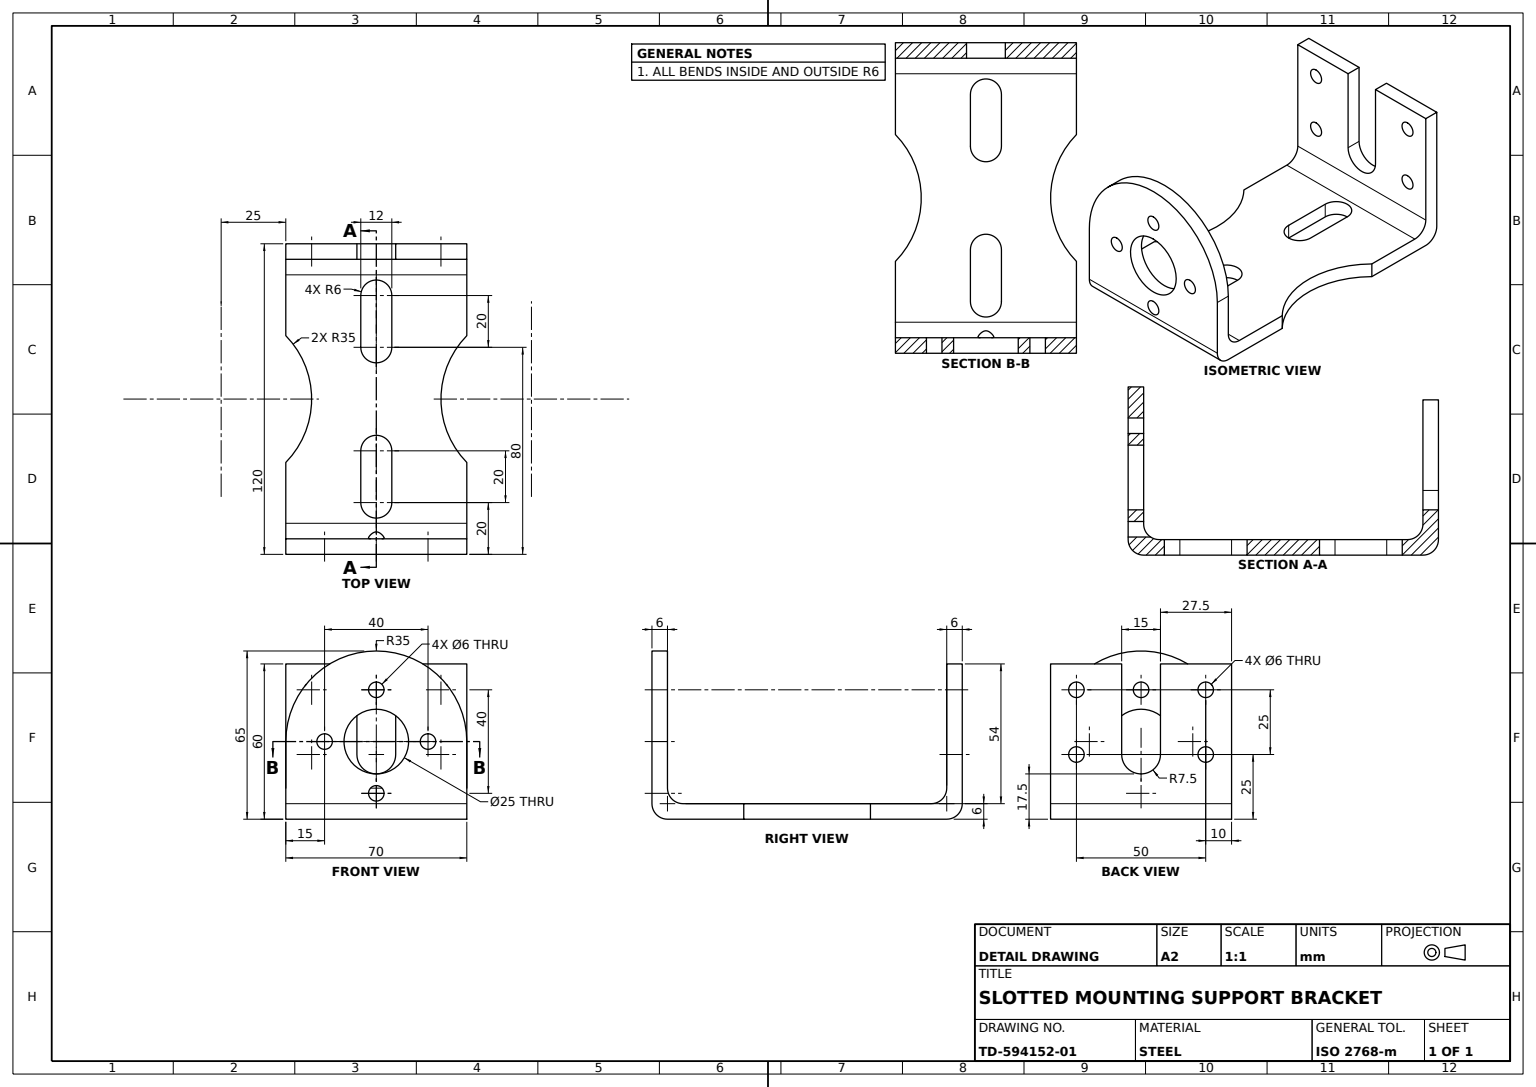
ISO-10303-21;
HEADER;
FILE_DESCRIPTION((''),'2;1');
FILE_NAME('','',(''),(''),'','','');
FILE_SCHEMA(('AUTOMOTIVE_DESIGN'));
ENDSEC;
DATA;
#1=APPLICATION_CONTEXT('');
#2=PRODUCT_CONTEXT('',#1,'mechanical');
#3=PRODUCT('','','',(#2));
#4=PRODUCT_DEFINITION_FORMATION('','',#3);
#5=PRODUCT_DEFINITION_CONTEXT('',#1,'design');
#6=PRODUCT_DEFINITION('','',#4,#5);
#7=PRODUCT_DEFINITION_SHAPE('','',#6);
#8=(LENGTH_UNIT()NAMED_UNIT(*)SI_UNIT(.MILLI.,.METRE.));
#9=(NAMED_UNIT(*)PLANE_ANGLE_UNIT()SI_UNIT($,.RADIAN.));
#10=(NAMED_UNIT(*)SI_UNIT($,.STERADIAN.)SOLID_ANGLE_UNIT());
#11=UNCERTAINTY_MEASURE_WITH_UNIT(LENGTH_MEASURE(0.005),#8,'distance_accuracy_value','');
#12=(GEOMETRIC_REPRESENTATION_CONTEXT(3)GLOBAL_UNCERTAINTY_ASSIGNED_CONTEXT((#11))GLOBAL_UNIT_ASSIGNED_CONTEXT((#8,#9,#10))REPRESENTATION_CONTEXT('',''));
#13=CARTESIAN_POINT('',(-54.,7.5,25.056417));
#14=VERTEX_POINT('',#13);
#15=CARTESIAN_POINT('',(-54.,-7.500212,25.));
#16=VERTEX_POINT('',#15);
#17=CARTESIAN_POINT('',(-54.,0.,25.));
#18=DIRECTION('',(1.,0.,0.));
#19=DIRECTION('',(0.,0.,-1.));
#20=AXIS2_PLACEMENT_3D('',#17,#18,#19);
#21=CIRCLE('',#20,7.500212);
#22=EDGE_CURVE('',#14,#16,#21,.F.);
#23=ORIENTED_EDGE('',*,*,#22,.F.);
#24=CARTESIAN_POINT('',(-60.,7.5,25.056417));
#25=VERTEX_POINT('',#24);
#26=CARTESIAN_POINT('',(-39.,7.5,25.056417));
#27=DIRECTION('',(-1.,0.,0.));
#28=VECTOR('',#27,1000.);
#29=LINE('',#26,#28);
#30=EDGE_CURVE('',#25,#14,#29,.F.);
#31=ORIENTED_EDGE('',*,*,#30,.F.);
#32=CARTESIAN_POINT('',(-60.,-7.500212,25.));
#33=VERTEX_POINT('',#32);
#34=CARTESIAN_POINT('',(-60.,0.,25.));
#35=AXIS2_PLACEMENT_3D('',#34,#18,#19);
#36=CIRCLE('',#35,7.500212);
#37=EDGE_CURVE('',#25,#33,#36,.F.);
#38=ORIENTED_EDGE('',*,*,#37,.T.);
#39=CARTESIAN_POINT('',(-39.,-7.500212,25.));
#40=LINE('',#39,#28);
#41=EDGE_CURVE('',#33,#16,#40,.F.);
#42=ORIENTED_EDGE('',*,*,#41,.T.);
#43=EDGE_LOOP('',(#23,#31,#38,#42));
#44=FACE_BOUND('',#43,.T.);
#45=CARTESIAN_POINT('',(-39.,0.,25.));
#46=DIRECTION('',(0.,0.,1.));
#47=AXIS2_PLACEMENT_3D('',#45,#27,#46);
#48=CYLINDRICAL_SURFACE('',#47,7.500212);
#49=ADVANCED_FACE('',(#44),#48,.F.);
#50=CARTESIAN_POINT('',(-54.,-7.500212,60.));
#51=VERTEX_POINT('',#50);
#52=CARTESIAN_POINT('',(-54.,-7.500212,0.));
#53=VECTOR('',#46,1000.);
#54=LINE('',#52,#53);
#55=EDGE_CURVE('',#16,#51,#54,.T.);
#56=ORIENTED_EDGE('',*,*,#55,.F.);
#57=ORIENTED_EDGE('',*,*,#41,.F.);
#58=CARTESIAN_POINT('',(-60.,-7.500212,60.));
#59=VERTEX_POINT('',#58);
#60=CARTESIAN_POINT('',(-60.,-7.500212,0.));
#61=LINE('',#60,#53);
#62=EDGE_CURVE('',#33,#59,#61,.T.);
#63=ORIENTED_EDGE('',*,*,#62,.T.);
#64=CARTESIAN_POINT('',(-39.,-7.500212,60.));
#65=LINE('',#64,#28);
#66=EDGE_CURVE('',#51,#59,#65,.T.);
#67=ORIENTED_EDGE('',*,*,#66,.F.);
#68=EDGE_LOOP('',(#56,#57,#63,#67));
#69=FACE_BOUND('',#68,.T.);
#70=DIRECTION('',(0.,1.,0.));
#71=AXIS2_PLACEMENT_3D('',#64,#70,#46);
#72=PLANE('',#71);
#73=ADVANCED_FACE('',(#69),#72,.T.);
#74=CARTESIAN_POINT('',(-20.,-6.,6.));
#75=VERTEX_POINT('',#74);
#76=CARTESIAN_POINT('',(-40.,-6.,6.));
#77=VERTEX_POINT('',#76);
#78=CARTESIAN_POINT('',(0.,-6.,6.));
#79=LINE('',#78,#28);
#80=EDGE_CURVE('',#75,#77,#79,.T.);
#81=ORIENTED_EDGE('',*,*,#80,.T.);
#82=CARTESIAN_POINT('',(-40.,6.,6.));
#83=VERTEX_POINT('',#82);
#84=CARTESIAN_POINT('',(-40.,0.,6.));
#85=AXIS2_PLACEMENT_3D('',#84,#19,#27);
#86=CIRCLE('',#85,6.);
#87=EDGE_CURVE('',#77,#83,#86,.T.);
#88=ORIENTED_EDGE('',*,*,#87,.T.);
#89=CARTESIAN_POINT('',(-20.,6.,6.));
#90=VERTEX_POINT('',#89);
#91=CARTESIAN_POINT('',(0.,6.,6.));
#92=VECTOR('',#18,1000.);
#93=LINE('',#91,#92);
#94=EDGE_CURVE('',#83,#90,#93,.T.);
#95=ORIENTED_EDGE('',*,*,#94,.T.);
#96=CARTESIAN_POINT('',(-20.,0.,6.));
#97=AXIS2_PLACEMENT_3D('',#96,#19,#27);
#98=CIRCLE('',#97,6.);
#99=EDGE_CURVE('',#90,#75,#98,.T.);
#100=ORIENTED_EDGE('',*,*,#99,.T.);
#101=EDGE_LOOP('',(#81,#88,#95,#100));
#102=FACE_BOUND('',#101,.T.);
#103=CARTESIAN_POINT('',(40.,6.,6.));
#104=VERTEX_POINT('',#103);
#105=CARTESIAN_POINT('',(20.,6.,6.));
#106=VERTEX_POINT('',#105);
#107=LINE('',#91,#28);
#108=EDGE_CURVE('',#104,#106,#107,.T.);
#109=ORIENTED_EDGE('',*,*,#108,.F.);
#110=CARTESIAN_POINT('',(40.,-6.,6.));
#111=VERTEX_POINT('',#110);
#112=CARTESIAN_POINT('',(40.,0.,6.));
#113=AXIS2_PLACEMENT_3D('',#112,#19,#27);
#114=CIRCLE('',#113,6.);
#115=EDGE_CURVE('',#111,#104,#114,.F.);
#116=ORIENTED_EDGE('',*,*,#115,.F.);
#117=CARTESIAN_POINT('',(20.,-6.,6.));
#118=VERTEX_POINT('',#117);
#119=LINE('',#78,#92);
#120=EDGE_CURVE('',#118,#111,#119,.T.);
#121=ORIENTED_EDGE('',*,*,#120,.F.);
#122=CARTESIAN_POINT('',(20.,0.,6.));
#123=AXIS2_PLACEMENT_3D('',#122,#19,#27);
#124=CIRCLE('',#123,6.);
#125=EDGE_CURVE('',#106,#118,#124,.F.);
#126=ORIENTED_EDGE('',*,*,#125,.F.);
#127=EDGE_LOOP('',(#109,#116,#121,#126));
#128=FACE_BOUND('',#127,.T.);
#129=CARTESIAN_POINT('',(48.,-35.,6.));
#130=VERTEX_POINT('',#129);
#131=CARTESIAN_POINT('',(24.494897,-35.,6.));
#132=VERTEX_POINT('',#131);
#133=CARTESIAN_POINT('',(60.,-35.,6.));
#134=LINE('',#133,#28);
#135=EDGE_CURVE('',#130,#132,#134,.T.);
#136=ORIENTED_EDGE('',*,*,#135,.F.);
#137=CARTESIAN_POINT('',(48.,35.,6.));
#138=VERTEX_POINT('',#137);
#139=DIRECTION('',(0.,-1.,0.));
#140=VECTOR('',#139,1000.);
#141=LINE('',#137,#140);
#142=EDGE_CURVE('',#130,#138,#141,.F.);
#143=ORIENTED_EDGE('',*,*,#142,.T.);
#144=CARTESIAN_POINT('',(24.494897,35.,6.));
#145=VERTEX_POINT('',#144);
#146=CARTESIAN_POINT('',(-60.,35.,6.));
#147=LINE('',#146,#92);
#148=EDGE_CURVE('',#145,#138,#147,.T.);
#149=ORIENTED_EDGE('',*,*,#148,.F.);
#150=CARTESIAN_POINT('',(-24.494897,35.,6.));
#151=VERTEX_POINT('',#150);
#152=CARTESIAN_POINT('',(0.,60.,6.));
#153=AXIS2_PLACEMENT_3D('',#152,#46,#18);
#154=CIRCLE('',#153,35.);
#155=EDGE_CURVE('',#151,#145,#154,.T.);
#156=ORIENTED_EDGE('',*,*,#155,.F.);
#157=CARTESIAN_POINT('',(-48.,35.,6.));
#158=VERTEX_POINT('',#157);
#159=EDGE_CURVE('',#158,#151,#147,.T.);
#160=ORIENTED_EDGE('',*,*,#159,.F.);
#161=CARTESIAN_POINT('',(-48.,-35.,6.));
#162=VERTEX_POINT('',#161);
#163=CARTESIAN_POINT('',(-48.,0.,6.));
#164=VECTOR('',#70,1000.);
#165=LINE('',#163,#164);
#166=EDGE_CURVE('',#158,#162,#165,.F.);
#167=ORIENTED_EDGE('',*,*,#166,.T.);
#168=CARTESIAN_POINT('',(-24.494897,-35.,6.));
#169=VERTEX_POINT('',#168);
#170=EDGE_CURVE('',#169,#162,#134,.T.);
#171=ORIENTED_EDGE('',*,*,#170,.F.);
#172=CARTESIAN_POINT('',(0.,-60.,6.));
#173=AXIS2_PLACEMENT_3D('',#172,#46,#18);
#174=CIRCLE('',#173,35.);
#175=EDGE_CURVE('',#132,#169,#174,.T.);
#176=ORIENTED_EDGE('',*,*,#175,.F.);
#177=EDGE_LOOP('',(#136,#143,#149,#156,#160,#167,#171,#176));
#178=FACE_BOUND('',#177,.T.);
#179=CARTESIAN_POINT('',(0.,0.,6.));
#180=AXIS2_PLACEMENT_3D('',#179,#19,#27);
#181=PLANE('',#180);
#182=ADVANCED_FACE('',(#102,#128,#178),#181,.F.);
#183=CARTESIAN_POINT('',(40.,6.,0.));
#184=VERTEX_POINT('',#183);
#185=CARTESIAN_POINT('',(40.,6.,-30.));
#186=LINE('',#185,#53);
#187=EDGE_CURVE('',#104,#184,#186,.F.);
#188=ORIENTED_EDGE('',*,*,#187,.T.);
#189=CARTESIAN_POINT('',(40.,-6.,0.));
#190=VERTEX_POINT('',#189);
#191=CARTESIAN_POINT('',(40.,0.,0.));
#192=AXIS2_PLACEMENT_3D('',#191,#46,#18);
#193=CIRCLE('',#192,6.);
#194=EDGE_CURVE('',#184,#190,#193,.F.);
#195=ORIENTED_EDGE('',*,*,#194,.T.);
#196=CARTESIAN_POINT('',(40.,-6.,-30.));
#197=LINE('',#196,#53);
#198=EDGE_CURVE('',#111,#190,#197,.F.);
#199=ORIENTED_EDGE('',*,*,#198,.F.);
#200=ORIENTED_EDGE('',*,*,#115,.T.);
#201=EDGE_LOOP('',(#188,#195,#199,#200));
#202=FACE_BOUND('',#201,.T.);
#203=CARTESIAN_POINT('',(40.,0.,-30.));
#204=AXIS2_PLACEMENT_3D('',#203,#46,#18);
#205=CYLINDRICAL_SURFACE('',#204,6.);
#206=ADVANCED_FACE('',(#202),#205,.F.);
#207=CARTESIAN_POINT('',(-20.,-6.,0.));
#208=VERTEX_POINT('',#207);
#209=CARTESIAN_POINT('',(-20.,-6.,-30.));
#210=LINE('',#209,#53);
#211=EDGE_CURVE('',#75,#208,#210,.F.);
#212=ORIENTED_EDGE('',*,*,#211,.T.);
#213=CARTESIAN_POINT('',(-40.,-6.,0.));
#214=VERTEX_POINT('',#213);
#215=CARTESIAN_POINT('',(-54.,-6.,0.));
#216=LINE('',#215,#92);
#217=EDGE_CURVE('',#214,#208,#216,.T.);
#218=ORIENTED_EDGE('',*,*,#217,.F.);
#219=CARTESIAN_POINT('',(-40.,-6.,-30.));
#220=LINE('',#219,#53);
#221=EDGE_CURVE('',#77,#214,#220,.F.);
#222=ORIENTED_EDGE('',*,*,#221,.F.);
#223=ORIENTED_EDGE('',*,*,#80,.F.);
#224=EDGE_LOOP('',(#212,#218,#222,#223));
#225=FACE_BOUND('',#224,.T.);
#226=AXIS2_PLACEMENT_3D('',#219,#139,#18);
#227=PLANE('',#226);
#228=ADVANCED_FACE('',(#225),#227,.F.);
#229=CARTESIAN_POINT('',(-54.,-25.,28.));
#230=VERTEX_POINT('',#229);
#231=CARTESIAN_POINT('',(-54.,-25.,25.));
#232=AXIS2_PLACEMENT_3D('',#231,#27,#46);
#233=CIRCLE('',#232,3.);
#234=EDGE_CURVE('',#230,#230,#233,.T.);
#235=ORIENTED_EDGE('',*,*,#234,.F.);
#236=EDGE_LOOP('',(#235));
#237=FACE_BOUND('',#236,.T.);
#238=CARTESIAN_POINT('',(-60.,-25.,22.));
#239=VERTEX_POINT('',#238);
#240=CARTESIAN_POINT('',(-60.,-25.,25.));
#241=AXIS2_PLACEMENT_3D('',#240,#18,#19);
#242=CIRCLE('',#241,3.);
#243=EDGE_CURVE('',#239,#239,#242,.T.);
#244=ORIENTED_EDGE('',*,*,#243,.F.);
#245=EDGE_LOOP('',(#244));
#246=FACE_BOUND('',#245,.T.);
#247=CYLINDRICAL_SURFACE('',#232,3.);
#248=ADVANCED_FACE('',(#237,#246),#247,.F.);
#249=CARTESIAN_POINT('',(20.,6.,0.));
#250=VERTEX_POINT('',#249);
#251=CARTESIAN_POINT('',(-54.,6.,0.));
#252=LINE('',#251,#92);
#253=EDGE_CURVE('',#250,#184,#252,.T.);
#254=ORIENTED_EDGE('',*,*,#253,.T.);
#255=ORIENTED_EDGE('',*,*,#187,.F.);
#256=ORIENTED_EDGE('',*,*,#108,.T.);
#257=CARTESIAN_POINT('',(20.,6.,-30.));
#258=LINE('',#257,#53);
#259=EDGE_CURVE('',#106,#250,#258,.F.);
#260=ORIENTED_EDGE('',*,*,#259,.T.);
#261=EDGE_LOOP('',(#254,#255,#256,#260));
#262=FACE_BOUND('',#261,.T.);
#263=AXIS2_PLACEMENT_3D('',#257,#139,#18);
#264=PLANE('',#263);
#265=ADVANCED_FACE('',(#262),#264,.T.);
#266=CARTESIAN_POINT('',(-60.,-25.,47.));
#267=VERTEX_POINT('',#266);
#268=CARTESIAN_POINT('',(-60.,-25.,50.));
#269=AXIS2_PLACEMENT_3D('',#268,#18,#19);
#270=CIRCLE('',#269,3.);
#271=EDGE_CURVE('',#267,#267,#270,.T.);
#272=ORIENTED_EDGE('',*,*,#271,.T.);
#273=EDGE_LOOP('',(#272));
#274=FACE_BOUND('',#273,.T.);
#275=CARTESIAN_POINT('',(-60.,25.,47.));
#276=VERTEX_POINT('',#275);
#277=CARTESIAN_POINT('',(-60.,25.,50.));
#278=AXIS2_PLACEMENT_3D('',#277,#18,#19);
#279=CIRCLE('',#278,3.);
#280=EDGE_CURVE('',#276,#276,#279,.T.);
#281=ORIENTED_EDGE('',*,*,#280,.T.);
#282=EDGE_LOOP('',(#281));
#283=FACE_BOUND('',#282,.T.);
#284=CARTESIAN_POINT('',(-60.,35.,60.));
#285=VERTEX_POINT('',#284);
#286=CARTESIAN_POINT('',(-60.,7.5,60.));
#287=VERTEX_POINT('',#286);
#288=LINE('',#284,#140);
#289=EDGE_CURVE('',#285,#287,#288,.T.);
#290=ORIENTED_EDGE('',*,*,#289,.F.);
#291=VERTEX_POINT('',#146);
#292=CARTESIAN_POINT('',(-60.,35.,0.));
#293=LINE('',#292,#53);
#294=EDGE_CURVE('',#285,#291,#293,.F.);
#295=ORIENTED_EDGE('',*,*,#294,.T.);
#296=CARTESIAN_POINT('',(-60.,-35.,6.));
#297=VERTEX_POINT('',#296);
#298=CARTESIAN_POINT('',(-60.,0.,6.));
#299=LINE('',#298,#164);
#300=EDGE_CURVE('',#291,#297,#299,.F.);
#301=ORIENTED_EDGE('',*,*,#300,.T.);
#302=CARTESIAN_POINT('',(-60.,-35.,60.));
#303=VERTEX_POINT('',#302);
#304=VECTOR('',#19,1000.);
#305=LINE('',#302,#304);
#306=EDGE_CURVE('',#303,#297,#305,.T.);
#307=ORIENTED_EDGE('',*,*,#306,.F.);
#308=EDGE_CURVE('',#59,#303,#288,.T.);
#309=ORIENTED_EDGE('',*,*,#308,.F.);
#310=ORIENTED_EDGE('',*,*,#62,.F.);
#311=ORIENTED_EDGE('',*,*,#37,.F.);
#312=CARTESIAN_POINT('',(-60.,7.5,0.));
#313=LINE('',#312,#304);
#314=EDGE_CURVE('',#287,#25,#313,.T.);
#315=ORIENTED_EDGE('',*,*,#314,.F.);
#316=EDGE_LOOP('',(#290,#295,#301,#307,#309,#310,#311,#315));
#317=FACE_BOUND('',#316,.T.);
#318=ORIENTED_EDGE('',*,*,#243,.T.);
#319=EDGE_LOOP('',(#318));
#320=FACE_BOUND('',#319,.T.);
#321=CARTESIAN_POINT('',(-60.,25.,22.));
#322=VERTEX_POINT('',#321);
#323=CARTESIAN_POINT('',(-60.,25.,25.));
#324=AXIS2_PLACEMENT_3D('',#323,#18,#19);
#325=CIRCLE('',#324,3.);
#326=EDGE_CURVE('',#322,#322,#325,.T.);
#327=ORIENTED_EDGE('',*,*,#326,.T.);
#328=EDGE_LOOP('',(#327));
#329=FACE_BOUND('',#328,.T.);
#330=CARTESIAN_POINT('',(-60.,0.,0.));
#331=AXIS2_PLACEMENT_3D('',#330,#18,#19);
#332=PLANE('',#331);
#333=ADVANCED_FACE('',(#274,#283,#317,#320,#329),#332,.F.);
#334=CARTESIAN_POINT('',(-54.,35.,12.));
#335=VERTEX_POINT('',#334);
#336=CARTESIAN_POINT('',(-54.,35.,60.));
#337=VERTEX_POINT('',#336);
#338=CARTESIAN_POINT('',(-54.,35.,0.));
#339=LINE('',#338,#53);
#340=EDGE_CURVE('',#335,#337,#339,.T.);
#341=ORIENTED_EDGE('',*,*,#340,.F.);
#342=CARTESIAN_POINT('',(-48.,35.,12.));
#343=AXIS2_PLACEMENT_3D('',#342,#139,#19);
#344=CIRCLE('',#343,6.);
#345=EDGE_CURVE('',#335,#158,#344,.T.);
#346=ORIENTED_EDGE('',*,*,#345,.T.);
#347=ORIENTED_EDGE('',*,*,#159,.T.);
#348=CARTESIAN_POINT('',(-24.494897,35.,0.));
#349=VERTEX_POINT('',#348);
#350=LINE('',#150,#304);
#351=EDGE_CURVE('',#349,#151,#350,.F.);
#352=ORIENTED_EDGE('',*,*,#351,.F.);
#353=VERTEX_POINT('',#338);
#354=LINE('',#338,#28);
#355=EDGE_CURVE('',#353,#349,#354,.F.);
#356=ORIENTED_EDGE('',*,*,#355,.F.);
#357=CARTESIAN_POINT('',(-54.,35.,6.));
#358=AXIS2_PLACEMENT_3D('',#357,#139,#19);
#359=CIRCLE('',#358,6.);
#360=EDGE_CURVE('',#353,#291,#359,.F.);
#361=ORIENTED_EDGE('',*,*,#360,.T.);
#362=ORIENTED_EDGE('',*,*,#294,.F.);
#363=LINE('',#336,#28);
#364=EDGE_CURVE('',#337,#285,#363,.T.);
#365=ORIENTED_EDGE('',*,*,#364,.F.);
#366=EDGE_LOOP('',(#341,#346,#347,#352,#356,#361,#362,#365));
#367=FACE_BOUND('',#366,.T.);
#368=AXIS2_PLACEMENT_3D('',#338,#139,#19);
#369=PLANE('',#368);
#370=ADVANCED_FACE('',(#367),#369,.F.);
#371=CARTESIAN_POINT('',(-54.,25.,53.));
#372=VERTEX_POINT('',#371);
#373=CARTESIAN_POINT('',(-54.,25.,50.));
#374=AXIS2_PLACEMENT_3D('',#373,#27,#46);
#375=CIRCLE('',#374,3.);
#376=EDGE_CURVE('',#372,#372,#375,.T.);
#377=ORIENTED_EDGE('',*,*,#376,.T.);
#378=EDGE_LOOP('',(#377));
#379=FACE_BOUND('',#378,.T.);
#380=CARTESIAN_POINT('',(-54.,25.,28.));
#381=VERTEX_POINT('',#380);
#382=CARTESIAN_POINT('',(-54.,25.,25.));
#383=AXIS2_PLACEMENT_3D('',#382,#27,#46);
#384=CIRCLE('',#383,3.);
#385=EDGE_CURVE('',#381,#381,#384,.T.);
#386=ORIENTED_EDGE('',*,*,#385,.T.);
#387=EDGE_LOOP('',(#386));
#388=FACE_BOUND('',#387,.T.);
#389=CARTESIAN_POINT('',(-54.,7.5,60.));
#390=VERTEX_POINT('',#389);
#391=LINE('',#336,#140);
#392=EDGE_CURVE('',#337,#390,#391,.T.);
#393=ORIENTED_EDGE('',*,*,#392,.T.);
#394=CARTESIAN_POINT('',(-54.,7.5,0.));
#395=LINE('',#394,#304);
#396=EDGE_CURVE('',#390,#14,#395,.T.);
#397=ORIENTED_EDGE('',*,*,#396,.T.);
#398=ORIENTED_EDGE('',*,*,#22,.T.);
#399=ORIENTED_EDGE('',*,*,#55,.T.);
#400=CARTESIAN_POINT('',(-54.,-35.,60.));
#401=VERTEX_POINT('',#400);
#402=EDGE_CURVE('',#51,#401,#391,.T.);
#403=ORIENTED_EDGE('',*,*,#402,.T.);
#404=CARTESIAN_POINT('',(-54.,-35.,12.));
#405=VERTEX_POINT('',#404);
#406=LINE('',#400,#304);
#407=EDGE_CURVE('',#401,#405,#406,.T.);
#408=ORIENTED_EDGE('',*,*,#407,.T.);
#409=CARTESIAN_POINT('',(-54.,0.,12.));
#410=LINE('',#409,#164);
#411=EDGE_CURVE('',#405,#335,#410,.T.);
#412=ORIENTED_EDGE('',*,*,#411,.T.);
#413=ORIENTED_EDGE('',*,*,#340,.T.);
#414=EDGE_LOOP('',(#393,#397,#398,#399,#403,#408,#412,#413));
#415=FACE_BOUND('',#414,.T.);
#416=ORIENTED_EDGE('',*,*,#234,.T.);
#417=EDGE_LOOP('',(#416));
#418=FACE_BOUND('',#417,.T.);
#419=CARTESIAN_POINT('',(-54.,-25.,53.));
#420=VERTEX_POINT('',#419);
#421=CARTESIAN_POINT('',(-54.,-25.,50.));
#422=AXIS2_PLACEMENT_3D('',#421,#27,#46);
#423=CIRCLE('',#422,3.);
#424=EDGE_CURVE('',#420,#420,#423,.T.);
#425=ORIENTED_EDGE('',*,*,#424,.T.);
#426=EDGE_LOOP('',(#425));
#427=FACE_BOUND('',#426,.T.);
#428=CARTESIAN_POINT('',(-54.,0.,0.));
#429=AXIS2_PLACEMENT_3D('',#428,#18,#19);
#430=PLANE('',#429);
#431=ADVANCED_FACE('',(#379,#388,#415,#418,#427),#430,.T.);
#432=CARTESIAN_POINT('',(54.,-2.236068,12.));
#433=VERTEX_POINT('',#432);
#434=CARTESIAN_POINT('',(54.,2.236068,12.));
#435=VERTEX_POINT('',#434);
#436=CARTESIAN_POINT('',(54.,-2.658422,11.527794));
#437=CARTESIAN_POINT('',(53.869214,-3.172061,10.315641));
#438=CARTESIAN_POINT('',(53.169965,-2.864386,8.857653));
#439=CARTESIAN_POINT('',(52.482087,-2.268413,7.985974));
#440=CARTESIAN_POINT('',(51.955003,-1.675796,7.470742));
#441=CARTESIAN_POINT('',(51.481666,-0.940993,7.106395));
#442=CARTESIAN_POINT('',(51.235187,-0.007069,6.947573));
#443=CARTESIAN_POINT('',(51.477387,0.934497,7.103347));
#444=CARTESIAN_POINT('',(51.953962,1.674353,7.469794));
#445=CARTESIAN_POINT('',(52.478961,2.26524,7.982636));
#446=CARTESIAN_POINT('',(53.168022,2.863317,8.854224));
#447=CARTESIAN_POINT('',(53.868442,3.172329,10.312555));
#448=CARTESIAN_POINT('',(54.,2.65991,11.52613));
#449=B_SPLINE_CURVE_WITH_KNOTS('',3,(#432,#436,#437,#438,#439,#440,#441,#442,#443,#444,#445,#446,#447,#448,#434),.UNSPECIFIED.,.F.,.F.,(4,1,1,1,1,1,1,1,1,1,1,1,4),(0.,0.001874522,0.003749044,0.004686305,0.005623566,0.006560827,0.007498087,0.008435348,0.009372609,0.01030987,0.011247131,0.013121653,0.014996175),.UNSPECIFIED.);
#450=EDGE_CURVE('',#433,#435,#449,.T.);
#451=ORIENTED_EDGE('',*,*,#450,.T.);
#452=CARTESIAN_POINT('',(54.,35.,12.));
#453=VERTEX_POINT('',#452);
#454=CARTESIAN_POINT('',(54.,-35.,12.));
#455=LINE('',#454,#140);
#456=EDGE_CURVE('',#453,#435,#455,.T.);
#457=ORIENTED_EDGE('',*,*,#456,.F.);
#458=CARTESIAN_POINT('',(48.,35.,12.));
#459=AXIS2_PLACEMENT_3D('',#458,#139,#19);
#460=CIRCLE('',#459,6.);
#461=EDGE_CURVE('',#138,#453,#460,.T.);
#462=ORIENTED_EDGE('',*,*,#461,.F.);
#463=ORIENTED_EDGE('',*,*,#142,.F.);
#464=VERTEX_POINT('',#454);
#465=CARTESIAN_POINT('',(48.,-35.,12.));
#466=AXIS2_PLACEMENT_3D('',#465,#70,#46);
#467=CIRCLE('',#466,6.);
#468=EDGE_CURVE('',#464,#130,#467,.T.);
#469=ORIENTED_EDGE('',*,*,#468,.F.);
#470=EDGE_CURVE('',#433,#464,#455,.T.);
#471=ORIENTED_EDGE('',*,*,#470,.F.);
#472=EDGE_LOOP('',(#451,#457,#462,#463,#469,#471));
#473=FACE_BOUND('',#472,.T.);
#474=CARTESIAN_POINT('',(48.,0.,12.));
#475=AXIS2_PLACEMENT_3D('',#474,#70,#46);
#476=CYLINDRICAL_SURFACE('',#475,6.);
#477=ADVANCED_FACE('',(#473),#476,.F.);
#478=CARTESIAN_POINT('',(-20.,6.,0.));
#479=VERTEX_POINT('',#478);
#480=CARTESIAN_POINT('',(-20.,0.,0.));
#481=AXIS2_PLACEMENT_3D('',#480,#46,#18);
#482=CIRCLE('',#481,6.);
#483=EDGE_CURVE('',#208,#479,#482,.T.);
#484=ORIENTED_EDGE('',*,*,#483,.F.);
#485=ORIENTED_EDGE('',*,*,#211,.F.);
#486=ORIENTED_EDGE('',*,*,#99,.F.);
#487=CARTESIAN_POINT('',(-20.,6.,-30.));
#488=LINE('',#487,#53);
#489=EDGE_CURVE('',#90,#479,#488,.F.);
#490=ORIENTED_EDGE('',*,*,#489,.T.);
#491=EDGE_LOOP('',(#484,#485,#486,#490));
#492=FACE_BOUND('',#491,.T.);
#493=CARTESIAN_POINT('',(-20.,0.,-30.));
#494=AXIS2_PLACEMENT_3D('',#493,#46,#18);
#495=CYLINDRICAL_SURFACE('',#494,6.);
#496=ADVANCED_FACE('',(#492),#495,.F.);
#497=ORIENTED_EDGE('',*,*,#326,.F.);
#498=EDGE_LOOP('',(#497));
#499=FACE_BOUND('',#498,.T.);
#500=ORIENTED_EDGE('',*,*,#385,.F.);
#501=EDGE_LOOP('',(#500));
#502=FACE_BOUND('',#501,.T.);
#503=CYLINDRICAL_SURFACE('',#383,3.);
#504=ADVANCED_FACE('',(#499,#502),#503,.F.);
#505=CARTESIAN_POINT('',(60.,-20.,33.));
#506=VERTEX_POINT('',#505);
#507=CARTESIAN_POINT('',(60.,-20.,30.));
#508=AXIS2_PLACEMENT_3D('',#507,#27,#46);
#509=CIRCLE('',#508,3.);
#510=EDGE_CURVE('',#506,#506,#509,.T.);
#511=ORIENTED_EDGE('',*,*,#510,.T.);
#512=EDGE_LOOP('',(#511));
#513=FACE_BOUND('',#512,.T.);
#514=CARTESIAN_POINT('',(60.,-35.,30.));
#515=VERTEX_POINT('',#514);
#516=VERTEX_POINT('',#133);
#517=LINE('',#133,#304);
#518=EDGE_CURVE('',#515,#516,#517,.T.);
#519=ORIENTED_EDGE('',*,*,#518,.T.);
#520=CARTESIAN_POINT('',(60.,35.,6.));
#521=VERTEX_POINT('',#520);
#522=LINE('',#520,#140);
#523=EDGE_CURVE('',#516,#521,#522,.F.);
#524=ORIENTED_EDGE('',*,*,#523,.T.);
#525=CARTESIAN_POINT('',(60.,35.,30.));
#526=VERTEX_POINT('',#525);
#527=LINE('',#520,#304);
#528=EDGE_CURVE('',#526,#521,#527,.T.);
#529=ORIENTED_EDGE('',*,*,#528,.F.);
#530=CARTESIAN_POINT('',(60.,0.,30.));
#531=AXIS2_PLACEMENT_3D('',#530,#18,#70);
#532=CIRCLE('',#531,35.);
#533=EDGE_CURVE('',#526,#515,#532,.T.);
#534=ORIENTED_EDGE('',*,*,#533,.T.);
#535=EDGE_LOOP('',(#519,#524,#529,#534));
#536=FACE_BOUND('',#535,.T.);
#537=CARTESIAN_POINT('',(60.,0.,13.));
#538=VERTEX_POINT('',#537);
#539=CARTESIAN_POINT('',(60.,0.,10.));
#540=AXIS2_PLACEMENT_3D('',#539,#27,#46);
#541=CIRCLE('',#540,3.);
#542=EDGE_CURVE('',#538,#538,#541,.T.);
#543=ORIENTED_EDGE('',*,*,#542,.T.);
#544=EDGE_LOOP('',(#543));
#545=FACE_BOUND('',#544,.T.);
#546=CARTESIAN_POINT('',(60.,0.,42.5));
#547=VERTEX_POINT('',#546);
#548=AXIS2_PLACEMENT_3D('',#530,#27,#46);
#549=CIRCLE('',#548,12.5);
#550=EDGE_CURVE('',#547,#547,#549,.T.);
#551=ORIENTED_EDGE('',*,*,#550,.T.);
#552=EDGE_LOOP('',(#551));
#553=FACE_BOUND('',#552,.T.);
#554=CARTESIAN_POINT('',(60.,0.,53.));
#555=VERTEX_POINT('',#554);
#556=CARTESIAN_POINT('',(60.,0.,50.));
#557=AXIS2_PLACEMENT_3D('',#556,#27,#46);
#558=CIRCLE('',#557,3.);
#559=EDGE_CURVE('',#555,#555,#558,.T.);
#560=ORIENTED_EDGE('',*,*,#559,.T.);
#561=EDGE_LOOP('',(#560));
#562=FACE_BOUND('',#561,.T.);
#563=CARTESIAN_POINT('',(60.,20.,33.));
#564=VERTEX_POINT('',#563);
#565=CARTESIAN_POINT('',(60.,20.,30.));
#566=AXIS2_PLACEMENT_3D('',#565,#27,#46);
#567=CIRCLE('',#566,3.);
#568=EDGE_CURVE('',#564,#564,#567,.T.);
#569=ORIENTED_EDGE('',*,*,#568,.T.);
#570=EDGE_LOOP('',(#569));
#571=FACE_BOUND('',#570,.T.);
#572=AXIS2_PLACEMENT_3D('',#520,#18,#19);
#573=PLANE('',#572);
#574=ADVANCED_FACE('',(#513,#536,#545,#553,#562,#571),#573,.T.);
#575=CARTESIAN_POINT('',(54.,-20.,27.));
#576=VERTEX_POINT('',#575);
#577=CARTESIAN_POINT('',(54.,-20.,30.));
#578=AXIS2_PLACEMENT_3D('',#577,#18,#19);
#579=CIRCLE('',#578,3.);
#580=EDGE_CURVE('',#576,#576,#579,.T.);
#581=ORIENTED_EDGE('',*,*,#580,.F.);
#582=EDGE_LOOP('',(#581));
#583=FACE_BOUND('',#582,.T.);
#584=ORIENTED_EDGE('',*,*,#510,.F.);
#585=EDGE_LOOP('',(#584));
#586=FACE_BOUND('',#585,.T.);
#587=CYLINDRICAL_SURFACE('',#508,3.);
#588=ADVANCED_FACE('',(#583,#586),#587,.F.);
#589=ORIENTED_EDGE('',*,*,#198,.T.);
#590=CARTESIAN_POINT('',(20.,-6.,0.));
#591=VERTEX_POINT('',#590);
#592=LINE('',#215,#28);
#593=EDGE_CURVE('',#190,#591,#592,.T.);
#594=ORIENTED_EDGE('',*,*,#593,.T.);
#595=CARTESIAN_POINT('',(20.,-6.,-30.));
#596=LINE('',#595,#53);
#597=EDGE_CURVE('',#118,#591,#596,.F.);
#598=ORIENTED_EDGE('',*,*,#597,.F.);
#599=ORIENTED_EDGE('',*,*,#120,.T.);
#600=EDGE_LOOP('',(#589,#594,#598,#599));
#601=FACE_BOUND('',#600,.T.);
#602=AXIS2_PLACEMENT_3D('',#196,#70,#27);
#603=PLANE('',#602);
#604=ADVANCED_FACE('',(#601),#603,.T.);
#605=ORIENTED_EDGE('',*,*,#300,.F.);
#606=ORIENTED_EDGE('',*,*,#360,.F.);
#607=CARTESIAN_POINT('',(-54.,-35.,0.));
#608=VERTEX_POINT('',#607);
#609=LINE('',#607,#164);
#610=EDGE_CURVE('',#608,#353,#609,.T.);
#611=ORIENTED_EDGE('',*,*,#610,.F.);
#612=CARTESIAN_POINT('',(-54.,-35.,6.));
#613=AXIS2_PLACEMENT_3D('',#612,#70,#46);
#614=CIRCLE('',#613,6.);
#615=EDGE_CURVE('',#297,#608,#614,.F.);
#616=ORIENTED_EDGE('',*,*,#615,.F.);
#617=EDGE_LOOP('',(#605,#606,#611,#616));
#618=FACE_BOUND('',#617,.T.);
#619=CYLINDRICAL_SURFACE('',#613,6.);
#620=ADVANCED_FACE('',(#618),#619,.T.);
#621=ORIENTED_EDGE('',*,*,#489,.F.);
#622=ORIENTED_EDGE('',*,*,#94,.F.);
#623=CARTESIAN_POINT('',(-40.,6.,0.));
#624=VERTEX_POINT('',#623);
#625=CARTESIAN_POINT('',(-40.,6.,-30.));
#626=LINE('',#625,#53);
#627=EDGE_CURVE('',#83,#624,#626,.F.);
#628=ORIENTED_EDGE('',*,*,#627,.T.);
#629=LINE('',#251,#28);
#630=EDGE_CURVE('',#479,#624,#629,.T.);
#631=ORIENTED_EDGE('',*,*,#630,.F.);
#632=EDGE_LOOP('',(#621,#622,#628,#631));
#633=FACE_BOUND('',#632,.T.);
#634=AXIS2_PLACEMENT_3D('',#487,#70,#27);
#635=PLANE('',#634);
#636=ADVANCED_FACE('',(#633),#635,.F.);
#637=ORIENTED_EDGE('',*,*,#424,.F.);
#638=EDGE_LOOP('',(#637));
#639=FACE_BOUND('',#638,.T.);
#640=ORIENTED_EDGE('',*,*,#271,.F.);
#641=EDGE_LOOP('',(#640));
#642=FACE_BOUND('',#641,.T.);
#643=CYLINDRICAL_SURFACE('',#422,3.);
#644=ADVANCED_FACE('',(#639,#642),#643,.F.);
#645=ORIENTED_EDGE('',*,*,#351,.T.);
#646=ORIENTED_EDGE('',*,*,#155,.T.);
#647=CARTESIAN_POINT('',(24.494897,35.,0.));
#648=VERTEX_POINT('',#647);
#649=LINE('',#144,#304);
#650=EDGE_CURVE('',#145,#648,#649,.T.);
#651=ORIENTED_EDGE('',*,*,#650,.T.);
#652=CARTESIAN_POINT('',(0.,60.,0.));
#653=AXIS2_PLACEMENT_3D('',#652,#46,#18);
#654=CIRCLE('',#653,35.);
#655=EDGE_CURVE('',#349,#648,#654,.T.);
#656=ORIENTED_EDGE('',*,*,#655,.F.);
#657=EDGE_LOOP('',(#645,#646,#651,#656));
#658=FACE_BOUND('',#657,.T.);
#659=AXIS2_PLACEMENT_3D('',#152,#19,#27);
#660=CYLINDRICAL_SURFACE('',#659,35.);
#661=ADVANCED_FACE('',(#658),#660,.F.);
#662=CARTESIAN_POINT('',(54.,20.,27.));
#663=VERTEX_POINT('',#662);
#664=CARTESIAN_POINT('',(54.,20.,30.));
#665=AXIS2_PLACEMENT_3D('',#664,#18,#19);
#666=CIRCLE('',#665,3.);
#667=EDGE_CURVE('',#663,#663,#666,.T.);
#668=ORIENTED_EDGE('',*,*,#667,.T.);
#669=EDGE_LOOP('',(#668));
#670=FACE_BOUND('',#669,.T.);
#671=CARTESIAN_POINT('',(54.,0.,17.5));
#672=VERTEX_POINT('',#671);
#673=CARTESIAN_POINT('',(54.,0.,30.));
#674=AXIS2_PLACEMENT_3D('',#673,#18,#19);
#675=CIRCLE('',#674,12.5);
#676=EDGE_CURVE('',#672,#672,#675,.T.);
#677=ORIENTED_EDGE('',*,*,#676,.T.);
#678=EDGE_LOOP('',(#677));
#679=FACE_BOUND('',#678,.T.);
#680=ORIENTED_EDGE('',*,*,#470,.T.);
#681=CARTESIAN_POINT('',(54.,-35.,30.));
#682=VERTEX_POINT('',#681);
#683=LINE('',#681,#304);
#684=EDGE_CURVE('',#682,#464,#683,.T.);
#685=ORIENTED_EDGE('',*,*,#684,.F.);
#686=CARTESIAN_POINT('',(54.,35.,30.));
#687=VERTEX_POINT('',#686);
#688=AXIS2_PLACEMENT_3D('',#673,#18,#70);
#689=CIRCLE('',#688,35.);
#690=EDGE_CURVE('',#687,#682,#689,.T.);
#691=ORIENTED_EDGE('',*,*,#690,.F.);
#692=CARTESIAN_POINT('',(54.,35.,0.));
#693=LINE('',#692,#53);
#694=EDGE_CURVE('',#453,#687,#693,.T.);
#695=ORIENTED_EDGE('',*,*,#694,.F.);
#696=ORIENTED_EDGE('',*,*,#456,.T.);
#697=CARTESIAN_POINT('',(54.,0.,10.));
#698=AXIS2_PLACEMENT_3D('',#697,#18,#19);
#699=CIRCLE('',#698,3.);
#700=EDGE_CURVE('',#435,#433,#699,.T.);
#701=ORIENTED_EDGE('',*,*,#700,.T.);
#702=EDGE_LOOP('',(#680,#685,#691,#695,#696,#701));
#703=FACE_BOUND('',#702,.T.);
#704=ORIENTED_EDGE('',*,*,#580,.T.);
#705=EDGE_LOOP('',(#704));
#706=FACE_BOUND('',#705,.T.);
#707=CARTESIAN_POINT('',(54.,0.,47.));
#708=VERTEX_POINT('',#707);
#709=CARTESIAN_POINT('',(54.,0.,50.));
#710=AXIS2_PLACEMENT_3D('',#709,#18,#19);
#711=CIRCLE('',#710,3.);
#712=EDGE_CURVE('',#708,#708,#711,.T.);
#713=ORIENTED_EDGE('',*,*,#712,.T.);
#714=EDGE_LOOP('',(#713));
#715=FACE_BOUND('',#714,.T.);
#716=PLANE('',#674);
#717=ADVANCED_FACE('',(#670,#679,#703,#706,#715),#716,.F.);
#718=ORIENTED_EDGE('',*,*,#650,.F.);
#719=ORIENTED_EDGE('',*,*,#148,.T.);
#720=ORIENTED_EDGE('',*,*,#461,.T.);
#721=ORIENTED_EDGE('',*,*,#694,.T.);
#722=LINE('',#686,#92);
#723=EDGE_CURVE('',#687,#526,#722,.T.);
#724=ORIENTED_EDGE('',*,*,#723,.T.);
#725=ORIENTED_EDGE('',*,*,#528,.T.);
#726=VERTEX_POINT('',#692);
#727=CARTESIAN_POINT('',(54.,35.,6.));
#728=AXIS2_PLACEMENT_3D('',#727,#139,#19);
#729=CIRCLE('',#728,6.);
#730=EDGE_CURVE('',#521,#726,#729,.F.);
#731=ORIENTED_EDGE('',*,*,#730,.T.);
#732=EDGE_CURVE('',#648,#726,#354,.F.);
#733=ORIENTED_EDGE('',*,*,#732,.F.);
#734=EDGE_LOOP('',(#718,#719,#720,#721,#724,#725,#731,#733));
#735=FACE_BOUND('',#734,.T.);
#736=ADVANCED_FACE('',(#735),#369,.F.);
#737=CARTESIAN_POINT('',(54.,-35.,0.));
#738=VERTEX_POINT('',#737);
#739=CARTESIAN_POINT('',(54.,-35.,6.));
#740=AXIS2_PLACEMENT_3D('',#739,#70,#46);
#741=CIRCLE('',#740,6.);
#742=EDGE_CURVE('',#738,#516,#741,.F.);
#743=ORIENTED_EDGE('',*,*,#742,.T.);
#744=ORIENTED_EDGE('',*,*,#518,.F.);
#745=LINE('',#681,#92);
#746=EDGE_CURVE('',#682,#515,#745,.T.);
#747=ORIENTED_EDGE('',*,*,#746,.F.);
#748=ORIENTED_EDGE('',*,*,#684,.T.);
#749=ORIENTED_EDGE('',*,*,#468,.T.);
#750=ORIENTED_EDGE('',*,*,#135,.T.);
#751=CARTESIAN_POINT('',(24.494897,-35.,0.));
#752=VERTEX_POINT('',#751);
#753=LINE('',#131,#304);
#754=EDGE_CURVE('',#752,#132,#753,.F.);
#755=ORIENTED_EDGE('',*,*,#754,.F.);
#756=LINE('',#607,#28);
#757=EDGE_CURVE('',#738,#752,#756,.T.);
#758=ORIENTED_EDGE('',*,*,#757,.F.);
#759=EDGE_LOOP('',(#743,#744,#747,#748,#749,#750,#755,#758));
#760=FACE_BOUND('',#759,.T.);
#761=AXIS2_PLACEMENT_3D('',#400,#70,#46);
#762=PLANE('',#761);
#763=ADVANCED_FACE('',(#760),#762,.F.);
#764=CARTESIAN_POINT('',(-40.,0.,0.));
#765=AXIS2_PLACEMENT_3D('',#764,#46,#18);
#766=CIRCLE('',#765,6.);
#767=EDGE_CURVE('',#624,#214,#766,.T.);
#768=ORIENTED_EDGE('',*,*,#767,.F.);
#769=ORIENTED_EDGE('',*,*,#627,.F.);
#770=ORIENTED_EDGE('',*,*,#87,.F.);
#771=ORIENTED_EDGE('',*,*,#221,.T.);
#772=EDGE_LOOP('',(#768,#769,#770,#771));
#773=FACE_BOUND('',#772,.T.);
#774=CARTESIAN_POINT('',(-40.,0.,-30.));
#775=AXIS2_PLACEMENT_3D('',#774,#46,#18);
#776=CYLINDRICAL_SURFACE('',#775,6.);
#777=ADVANCED_FACE('',(#773),#776,.F.);
#778=ORIENTED_EDGE('',*,*,#450,.F.);
#779=ORIENTED_EDGE('',*,*,#700,.F.);
#780=EDGE_LOOP('',(#778,#779));
#781=FACE_BOUND('',#780,.T.);
#782=ORIENTED_EDGE('',*,*,#542,.F.);
#783=EDGE_LOOP('',(#782));
#784=FACE_BOUND('',#783,.T.);
#785=CYLINDRICAL_SURFACE('',#540,3.);
#786=ADVANCED_FACE('',(#781,#784),#785,.F.);
#787=ORIENTED_EDGE('',*,*,#667,.F.);
#788=EDGE_LOOP('',(#787));
#789=FACE_BOUND('',#788,.T.);
#790=ORIENTED_EDGE('',*,*,#568,.F.);
#791=EDGE_LOOP('',(#790));
#792=FACE_BOUND('',#791,.T.);
#793=CYLINDRICAL_SURFACE('',#566,3.);
#794=ADVANCED_FACE('',(#789,#792),#793,.F.);
#795=ORIENTED_EDGE('',*,*,#175,.T.);
#796=CARTESIAN_POINT('',(-24.494897,-35.,0.));
#797=VERTEX_POINT('',#796);
#798=LINE('',#168,#304);
#799=EDGE_CURVE('',#169,#797,#798,.T.);
#800=ORIENTED_EDGE('',*,*,#799,.T.);
#801=CARTESIAN_POINT('',(0.,-60.,0.));
#802=AXIS2_PLACEMENT_3D('',#801,#46,#18);
#803=CIRCLE('',#802,35.);
#804=EDGE_CURVE('',#752,#797,#803,.T.);
#805=ORIENTED_EDGE('',*,*,#804,.F.);
#806=ORIENTED_EDGE('',*,*,#754,.T.);
#807=EDGE_LOOP('',(#795,#800,#805,#806));
#808=FACE_BOUND('',#807,.T.);
#809=AXIS2_PLACEMENT_3D('',#172,#19,#27);
#810=CYLINDRICAL_SURFACE('',#809,35.);
#811=ADVANCED_FACE('',(#808),#810,.F.);
#812=ORIENTED_EDGE('',*,*,#30,.T.);
#813=ORIENTED_EDGE('',*,*,#396,.F.);
#814=CARTESIAN_POINT('',(-39.,7.5,60.));
#815=LINE('',#814,#28);
#816=EDGE_CURVE('',#390,#287,#815,.T.);
#817=ORIENTED_EDGE('',*,*,#816,.T.);
#818=ORIENTED_EDGE('',*,*,#314,.T.);
#819=EDGE_LOOP('',(#812,#813,#817,#818));
#820=FACE_BOUND('',#819,.T.);
#821=AXIS2_PLACEMENT_3D('',#26,#139,#19);
#822=PLANE('',#821);
#823=ADVANCED_FACE('',(#820),#822,.T.);
#824=ORIENTED_EDGE('',*,*,#690,.T.);
#825=ORIENTED_EDGE('',*,*,#746,.T.);
#826=ORIENTED_EDGE('',*,*,#533,.F.);
#827=ORIENTED_EDGE('',*,*,#723,.F.);
#828=EDGE_LOOP('',(#824,#825,#826,#827));
#829=FACE_BOUND('',#828,.T.);
#830=CYLINDRICAL_SURFACE('',#674,35.);
#831=ADVANCED_FACE('',(#829),#830,.T.);
#832=ORIENTED_EDGE('',*,*,#550,.F.);
#833=EDGE_LOOP('',(#832));
#834=FACE_BOUND('',#833,.T.);
#835=ORIENTED_EDGE('',*,*,#676,.F.);
#836=EDGE_LOOP('',(#835));
#837=FACE_BOUND('',#836,.T.);
#838=CYLINDRICAL_SURFACE('',#548,12.5);
#839=ADVANCED_FACE('',(#834,#837),#838,.F.);
#840=CARTESIAN_POINT('',(20.,0.,0.));
#841=AXIS2_PLACEMENT_3D('',#840,#46,#18);
#842=CIRCLE('',#841,6.);
#843=EDGE_CURVE('',#591,#250,#842,.F.);
#844=ORIENTED_EDGE('',*,*,#843,.F.);
#845=ORIENTED_EDGE('',*,*,#593,.F.);
#846=ORIENTED_EDGE('',*,*,#194,.F.);
#847=ORIENTED_EDGE('',*,*,#253,.F.);
#848=EDGE_LOOP('',(#844,#845,#846,#847));
#849=FACE_BOUND('',#848,.T.);
#850=ORIENTED_EDGE('',*,*,#767,.T.);
#851=ORIENTED_EDGE('',*,*,#217,.T.);
#852=ORIENTED_EDGE('',*,*,#483,.T.);
#853=ORIENTED_EDGE('',*,*,#630,.T.);
#854=EDGE_LOOP('',(#850,#851,#852,#853));
#855=FACE_BOUND('',#854,.T.);
#856=EDGE_CURVE('',#797,#608,#756,.T.);
#857=ORIENTED_EDGE('',*,*,#856,.T.);
#858=ORIENTED_EDGE('',*,*,#610,.T.);
#859=ORIENTED_EDGE('',*,*,#355,.T.);
#860=ORIENTED_EDGE('',*,*,#655,.T.);
#861=ORIENTED_EDGE('',*,*,#732,.T.);
#862=LINE('',#737,#140);
#863=EDGE_CURVE('',#726,#738,#862,.T.);
#864=ORIENTED_EDGE('',*,*,#863,.T.);
#865=ORIENTED_EDGE('',*,*,#757,.T.);
#866=ORIENTED_EDGE('',*,*,#804,.T.);
#867=EDGE_LOOP('',(#857,#858,#859,#860,#861,#864,#865,#866));
#868=FACE_BOUND('',#867,.T.);
#869=AXIS2_PLACEMENT_3D('',#607,#46,#18);
#870=PLANE('',#869);
#871=ADVANCED_FACE('',(#849,#855,#868),#870,.F.);
#872=ORIENTED_EDGE('',*,*,#816,.F.);
#873=ORIENTED_EDGE('',*,*,#392,.F.);
#874=ORIENTED_EDGE('',*,*,#364,.T.);
#875=ORIENTED_EDGE('',*,*,#289,.T.);
#876=EDGE_LOOP('',(#872,#873,#874,#875));
#877=FACE_BOUND('',#876,.T.);
#878=AXIS2_PLACEMENT_3D('',#336,#19,#27);
#879=PLANE('',#878);
#880=ADVANCED_FACE('',(#877),#879,.F.);
#881=ORIENTED_EDGE('',*,*,#166,.F.);
#882=ORIENTED_EDGE('',*,*,#345,.F.);
#883=ORIENTED_EDGE('',*,*,#411,.F.);
#884=CARTESIAN_POINT('',(-48.,-35.,12.));
#885=AXIS2_PLACEMENT_3D('',#884,#70,#46);
#886=CIRCLE('',#885,6.);
#887=EDGE_CURVE('',#162,#405,#886,.T.);
#888=ORIENTED_EDGE('',*,*,#887,.F.);
#889=EDGE_LOOP('',(#881,#882,#883,#888));
#890=FACE_BOUND('',#889,.T.);
#891=CARTESIAN_POINT('',(-48.,0.,12.));
#892=AXIS2_PLACEMENT_3D('',#891,#70,#46);
#893=CYLINDRICAL_SURFACE('',#892,6.);
#894=ADVANCED_FACE('',(#890),#893,.F.);
#895=ORIENTED_EDGE('',*,*,#66,.T.);
#896=ORIENTED_EDGE('',*,*,#308,.T.);
#897=LINE('',#400,#28);
#898=EDGE_CURVE('',#401,#303,#897,.T.);
#899=ORIENTED_EDGE('',*,*,#898,.F.);
#900=ORIENTED_EDGE('',*,*,#402,.F.);
#901=EDGE_LOOP('',(#895,#896,#899,#900));
#902=FACE_BOUND('',#901,.T.);
#903=ADVANCED_FACE('',(#902),#879,.F.);
#904=ORIENTED_EDGE('',*,*,#280,.F.);
#905=EDGE_LOOP('',(#904));
#906=FACE_BOUND('',#905,.T.);
#907=ORIENTED_EDGE('',*,*,#376,.F.);
#908=EDGE_LOOP('',(#907));
#909=FACE_BOUND('',#908,.T.);
#910=CYLINDRICAL_SURFACE('',#374,3.);
#911=ADVANCED_FACE('',(#906,#909),#910,.F.);
#912=ORIENTED_EDGE('',*,*,#125,.T.);
#913=ORIENTED_EDGE('',*,*,#597,.T.);
#914=ORIENTED_EDGE('',*,*,#843,.T.);
#915=ORIENTED_EDGE('',*,*,#259,.F.);
#916=EDGE_LOOP('',(#912,#913,#914,#915));
#917=FACE_BOUND('',#916,.T.);
#918=CARTESIAN_POINT('',(20.,0.,-30.));
#919=AXIS2_PLACEMENT_3D('',#918,#46,#18);
#920=CYLINDRICAL_SURFACE('',#919,6.);
#921=ADVANCED_FACE('',(#917),#920,.F.);
#922=ORIENTED_EDGE('',*,*,#712,.F.);
#923=EDGE_LOOP('',(#922));
#924=FACE_BOUND('',#923,.T.);
#925=ORIENTED_EDGE('',*,*,#559,.F.);
#926=EDGE_LOOP('',(#925));
#927=FACE_BOUND('',#926,.T.);
#928=CYLINDRICAL_SURFACE('',#557,3.);
#929=ADVANCED_FACE('',(#924,#927),#928,.F.);
#930=ORIENTED_EDGE('',*,*,#742,.F.);
#931=ORIENTED_EDGE('',*,*,#863,.F.);
#932=ORIENTED_EDGE('',*,*,#730,.F.);
#933=ORIENTED_EDGE('',*,*,#523,.F.);
#934=EDGE_LOOP('',(#930,#931,#932,#933));
#935=FACE_BOUND('',#934,.T.);
#936=CYLINDRICAL_SURFACE('',#740,6.);
#937=ADVANCED_FACE('',(#935),#936,.T.);
#938=ORIENTED_EDGE('',*,*,#170,.T.);
#939=ORIENTED_EDGE('',*,*,#887,.T.);
#940=ORIENTED_EDGE('',*,*,#407,.F.);
#941=ORIENTED_EDGE('',*,*,#898,.T.);
#942=ORIENTED_EDGE('',*,*,#306,.T.);
#943=ORIENTED_EDGE('',*,*,#615,.T.);
#944=ORIENTED_EDGE('',*,*,#856,.F.);
#945=ORIENTED_EDGE('',*,*,#799,.F.);
#946=EDGE_LOOP('',(#938,#939,#940,#941,#942,#943,#944,#945));
#947=FACE_BOUND('',#946,.T.);
#948=ADVANCED_FACE('',(#947),#762,.F.);
#949=CLOSED_SHELL('',(#49,#73,#182,#206,#228,#248,#265,#333,#370,#431,#477,#496,#504,#574,#588,#604,#620,#636,#644,#661,#717,#736,#763,#777,#786,#794,#811,#823,#831,#839,#871,#880,#894,#903,#911,#921,#929,#937,#948));
#950=MANIFOLD_SOLID_BREP('',#949);
#951=ADVANCED_BREP_SHAPE_REPRESENTATION('',(#950),#12);
#952=SHAPE_DEFINITION_REPRESENTATION(#7,#951);
ENDSEC;
END-ISO-10303-21;
